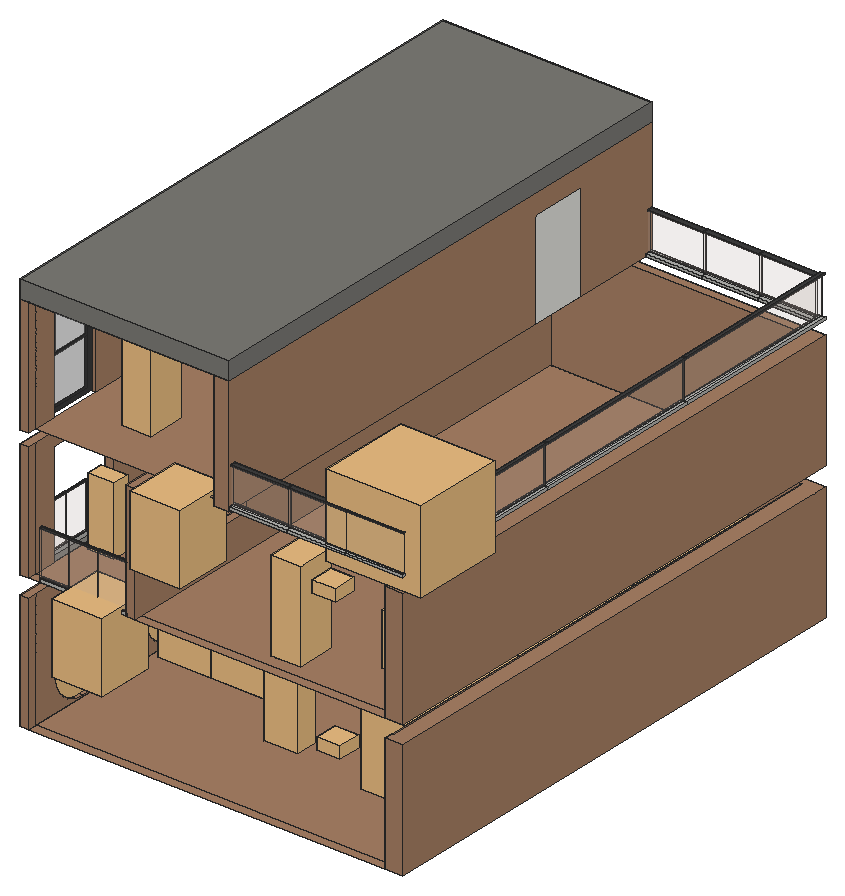
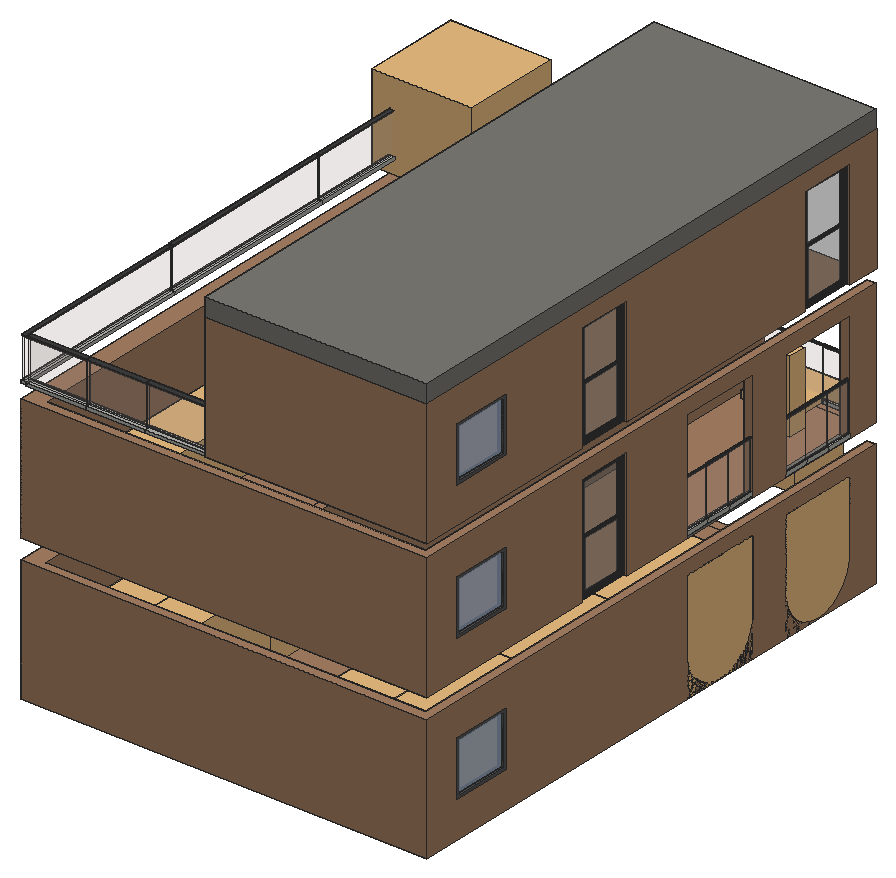
# SketchUp Ruby script. Lengths in inches.
U = 1.inch
M = Sketchup.active_model
def pt(a) = Geom::Point3d.new(a.map { |v| v * U })
def face(e, loops, mat)
  f = e.add_face(loops[0].map { |a| pt(a) })
  loops[1..].each { |l| e.add_face(l.map { |a| pt(a) }).erase! }
  f.material = f.back_material = mat if mat
  f
end
# faces: each face lists its corners as indices into pts; further lists are holes
def faces(e, pts, list, mat = nil) = list.each { |f| face(e, (f[0].is_a?(Array) ? f : [f]).map { |l| l.map { |i| pts[i] } }, mat) }
# xy, xz, yz: faces in a plane at the given z, y or x. An outline is a flat list of corners, or four numbers for a rectangle; further outlines are holes
def ring(l) = l.size == 4 ? [[l[0], l[1]], [l[2], l[1]], [l[2], l[3]], [l[0], l[3]]] : l.each_slice(2).to_a
def flat(e, list, mat, &to3) = list.each { |f| face(e, (f[0].is_a?(Array) ? f : [f]).map { |l| ring(l).map { |u, v| to3.(u, v) } }, mat) }
def xy(e, z, list, mat = nil) = flat(e, list, mat) { |x, y| [x, y, z] }
def xz(e, y, list, mat = nil) = flat(e, list, mat) { |x, z| [x, y, z] }
def yz(e, x, list, mat = nil) = flat(e, list, mat) { |y, z| [x, y, z] }
def lines(e, pts, list) = list.each { |a, b| e.add_line(pt(pts[a]), pt(pts[b])) }
# prism: a flat outline (further loops are holes) pulled along v
def prism(e, loops, v, mat = nil)
  f = face(e, loops, mat); d = Geom::Vector3d.new(v.map { |x| x * U })
  f.pushpull(f.normal.samedirection?(d) ? d.length : -d.length)
end
def box(e, o, s, mat = nil) = prism(e, [[o, [o[0] + s[0], o[1], o[2]], [o[0] + s[0], o[1] + s[1], o[2]], [o[0], o[1] + s[1], o[2]]]], [0, 0, s[2]], mat)
def at(x, y, z, deg = 0) = Geom::Transformation.translation(pt([x, y, z])) * Geom::Transformation.rotation(ORIGIN, Z_AXIS, deg.degrees)
def axes(o, x, y, z) = Geom::Transformation.new([*x, 0, *y, 0, *z, 0, *pt(o).to_a, 1])
def part(name) = M.definitions.add(name)
# library, detail: a bought-in or finely detailed component or shape, given as its bounding box
def library(name, o, s) = part(name).tap { |d| box(d.entities, o, s) }
def detail(e, o, s) = box(e.add_group.entities, o, s)
def put(e, d, t, mat = nil) = e.add_instance(d, t).tap { |i| i.material = mat if mat }
def group(e, t, mat = nil) = e.add_group.tap { |g| g.transformation = t; g.material = mat if mat }.entities
root = M.entities
M.materials.add("Aluminum_Anodized_Clear\#1").color = [178, 178, 174]
M.materials.add("Aluminum_Anodized_DarkGray\#1").color = [63, 63, 63]
M.materials.add("Bricks A04 100cm").color = [167, 128, 100]
M.materials.add("Concrete Grey 06 100cm").color = [123, 122, 117]
M.materials.add("Windows").color = [58, 58, 58]
M.materials.add("[Color_006]").color = [86, 86, 86]
M.materials.add("[Translucent Glass Gray]1").color = [128, 128, 128]
M.materials["[Translucent Glass Gray]1"].alpha = 0.5
M.materials.add("[Translucent_Glass_Gray]").color = [128, 128, 128]
M.materials["[Translucent_Glass_Gray]"].alpha = 0.5
M.materials.add("[Translucent_Glass_Gray]1").color = [167, 187, 214]
M.materials["[Translucent_Glass_Gray]1"].alpha = 0.8
M.materials.add("glass_architectural\#1").color = [217, 197, 188]
M.materials["glass_architectural\#1"].alpha = 0.1
c1 = library("Tariq 001 Standing",[-13.52,-8.8,0],[27.07,17.52,69.71])
c2 = library("Group\#170",[0,0,-0.09],[44.81,94.49,48.85])
c3 = library("Group\#172",[0,0,-0.09],[44.81,94.49,48.85])
c4 = part("Office workstation bank")
put(c4.entities,c2,at(188.98,44.81,0.09,-90))
put(c4.entities,c3,axes([0,44.81,0.09],[0,1,0],[1,0,0],[0,0,1]))
put(c4.entities,c3,axes([188.98,44.81,0.09],[0,1,0],[1,0,0],[0,0,1]))
put(c4.entities,c2,at(0,44.81,0.09,-90))
put(c4.entities,c2,at(94.49,44.81,0.09,-90))
put(c4.entities,c3,axes([94.49,44.81,0.09],[0,1,0],[1,0,0],[0,0,1]))
c5 = library("Group\#17",[0,0,0],[177.17,118.11,3.9375])
c6 = part("window+1")
g1 = group(c6.entities,at(0,0,177.17))
put(g1,c5,axes([0,0,0],[0,0,-1],[0,1,0],[1,0,0]))
g2 = group(g1,at(1.97,3.9375,-4.36),"[Translucent_Glass_Gray]")
yz(g2,0,[[0,-168.87,26.65,-142.34],[28.62,-168.87,51.08,-142.34],[59.15,-168.87,81.32,-142.34],[83.29,-168.87,110.24,-142.34],[0,-140.375,26.65,-114.83],
  [28.62,-140.375,51.08,-114.83],[59.15,-140.375,81.32,-114.83],[83.29,-140.375,110.24,-114.83],[0,-112.86,26.65,-87.32],[28.62,-112.86,51.08,-87.32],
  [59.15,-112.86,81.32,-87.32],[83.29,-112.86,110.24,-87.32],[0,-85.35,26.65,-58.83],[28.62,-85.35,51.08,-58.83],[59.15,-85.35,81.32,-58.83],
  [83.29,-85.35,110.24,-58.83],[0.55,-50.76,26.65,-50.76,26.93,-47.45,27.62,-44.2,28.72,-41.07,30.21,-38.1,32.07,-35.35,33.61,-33.59,15.58,-16.55,15.5625,-16.53,7.41,-27.15,1.91,-40.4375],[28.79,-50.76,52.17,-50.76,52.17,-27.38,50.2,-27.38,49.14,-27.47,46.14,-28.11,43.24,-29.125,40.5,-30.5,37.96,-32.22,35.65,-34.25,33.63,-36.55,31.91,-39.1,30.53,-41.84,29.52,-44.73,28.875,-47.74,28.79,-48.79],[58.07,-50.76,81.32,-50.76,81.32,-48.79,81.24,-47.74,80.61,-44.75,79.6,-41.87,78.24,-39.14,76.53,-36.61,74.52,-34.3125,72.22,-32.3,69.6875,-30.59,66.96,-29.22,64.08,-28.22,61.09,-27.59,60.04,-27.51,58.07,-27.51],[83.45,-50.76,109.68,-50.76,108.33,-40.4375,102.82,-27.15,94.67,-16.53,76.5625,-33.66,78.09,-35.4,79.94,-38.15,81.42,-41.1,82.51,-44.23,83.19,-47.46],
  [75.17,-32.27,93.28,-15.14,82.66,-6.99,69.375,-1.49,58.07,0,58.07,-25.38,61.37,-25.64,64.6,-26.32,67.73,-27.41,70.68,-28.89,73.43,-30.74],[35,-32.2,36.75,-30.66,39.51,-28.8,42.47,-27.31,45.61,-26.21,48.86,-25.52,52.17,-25.25,52.17,0,40.86,-1.49,27.58,-6.99,16.96,-15.14]])
put(g1,c5,axes([0,182.58,0],[0,0,-1],[0,1,0],[1,0,0]))
c7 = part("BIC_Bike Shop - Window - Small")
xy(c7.entities,-8,[[[0,0,36,36],[2,2,34,34]]],"[Color_006]")
xy(c7.entities,-4,[[2,2,34,34]],"[Translucent_Glass_Gray]1")
xy(c7.entities,0,[[[0,0,36,36],[2,2,34,34]]],"[Color_006]")
xz(c7.entities,0,[[0,-8,36,0]],"[Color_006]")
xz(c7.entities,2,[[2,-8,34,-4],[2,-4,34,0]],"[Color_006]")
xz(c7.entities,34,[[2,-8,34,-4],[2,-4,34,0]],"[Color_006]")
xz(c7.entities,36,[[0,-8,36,0]],"[Color_006]")
yz(c7.entities,0,[[0,-8,36,0]],"[Color_006]")
yz(c7.entities,2,[[2,-8,34,-4],[2,-4,34,0]],"[Color_006]")
yz(c7.entities,34,[[2,-8,34,-4],[2,-4,34,0]],"[Color_006]")
yz(c7.entities,36,[[0,-8,36,0]],"[Color_006]")
c8 = library("Untitled+(35)",[-36.2,-34.81,25.37],[51.5,58.42,71.3])
c9 = library("Dome Light",[-12,-12,0],[24,24,12])
c10 = part("Window+06")
g3 = group(c10.entities,at(-11,5.5,0,-90))
xy(g3,0,[[0,11,5.5,35]],"Windows")
xy(g3,2,[[0,13,5.5,33]],"Windows")
xy(g3,53,[[0,13,5.5,33]],"Windows")
xy(g3,55,[[0,11,5.5,35]],"Windows")
xz(g3,11,[[0,0,5.5,55]],"Windows")
xz(g3,13,[[0,2,5.5,53]],"Windows")
xz(g3,33,[[0,2,5.5,53]],"Windows")
xz(g3,35,[[0,0,5.5,55]],"Windows")
yz(g3,0,[[[11,0,35,55],[13,2,33,53]]],"Windows")
yz(g3,5.5,[[[11,0,35,55],[13,2,33,53]]],"Windows")
g4 = group(g3,at(2.75,2,2))
xy(g4,0,[[0,11,2,31]],"Windows")
xy(g4,1,[[0,12,1,30],[1,12,2,30]],"Windows")
xy(g4,25,[[0,12,1,30],[1,12,2,30]],"Windows")
xy(g4,26,[[0,11,2,31]],"Windows")
xz(g4,11,[[0,0,2,26]],"Windows")
xz(g4,12,[[0,1,1,25],[1,1,2,25]],"Windows")
xz(g4,30,[[0,1,1,25],[1,1,2,25]],"Windows")
xz(g4,31,[[0,0,2,26]],"Windows")
yz(g4,0,[[[11,0,31,26],[12,1,30,25]]],"Windows")
yz(g4,1,[[12,1,30,25]],"[Translucent Glass Gray]1")
yz(g4,2,[[[11,0,31,26],[12,1,30,25]]],"Windows")
g5 = group(g3,at(0.75,2,27))
xy(g5,0,[[0,11,2,31]],"Windows")
xy(g5,1,[[0,12,1,30],[1,12,2,30]],"Windows")
xy(g5,25,[[0,12,1,30],[1,12,2,30]],"Windows")
xy(g5,26,[[0,11,2,31]],"Windows")
xz(g5,11,[[0,0,2,26]],"Windows")
xz(g5,12,[[0,1,1,25],[1,1,2,25]],"Windows")
xz(g5,30,[[0,1,1,25],[1,1,2,25]],"Windows")
xz(g5,31,[[0,0,2,26]],"Windows")
yz(g5,0,[[[11,0,31,26],[12,1,30,25]]],"Windows")
yz(g5,1,[[12,1,30,25]],"[Translucent Glass Gray]1")
yz(g5,2,[[[11,0,31,26],[12,1,30,25]]],"Windows")
c11 = library("Reception desk",[23.57,0,0],[37.45,80.71,54.72])
c12 = library("Katja 001 Standing",[-10.51,-13.65,0],[20.97,27.3,64.32])
c13 = part("GLASS")
prism(c13.entities,[[[48,0,0],[0,0,0],[0,0.8,0],[48.96,0.8,0]]],[0,0,36])
c14 = part("STEEL BAR")
box(c14.entities,[0,-0.1,0],[48,1.8,1.2])
c15 = part("LOWER PART")
box(c15.entities,[0,-0.6,0],[48.6,2.6,2.6])
c16 = part("BALCONY GLASS ")
put(c16.entities,c13,at(0,0.9,2.6),"glass_architectural\#1")
put(c16.entities,c14,at(0,0.5,38.6),"Aluminum_Anodized_DarkGray\#1")
put(c16.entities,c15,at(0,0.6,0),"Aluminum_Anodized_Clear\#1")
c17 = part("NO 3")
put(c17.entities,c16,at(0,0,0))
put(c17.entities,c16,at(48.6,0,0))
put(c17.entities,c16,at(97.2,0,0))
c18 = library("Dome Light\#1",[-12,-12,0],[24,24,12])
c19 = library("Palmilla",[-52.93,-43.2,-6.65],[96.66,94.88,84.22])
box(root,[396.25,532.6875,414.5625],[57.5625,56.26,98.76])
xy(root,281.8125,[[240.0625,289.51,249.0625,368.7]])
xy(root,282.82,[[240.0625,173.32,249.0625,249.35]],"Concrete Grey 06 100cm")
xy(root,283.0625,[[240.0625,289.51,249.0625,368.7]])
xz(root,289.51,[[240.0625,281.8125,249.0625,283.0625]])
xz(root,368.7,[[240.0625,281.8125,249.0625,283.0625]])
yz(root,240.0625,[[173.32,281.8125,173.32,282.82,249.35,282.82,252.52,281.8125],[289.51,281.8125,368.7,283.0625]],"Concrete Grey 06 100cm")
yz(root,249.0625,[[289.51,281.8125,368.7,283.0625]])
put(root,c1,axes([423.48,256.09,142.06],[1.25,0,0],[0,1.25,0],[0,0,1.25]))
put(root,c4,axes([516.21,672.11,142.85],[0,-1.55368,0],[1,0,0],[0,0,1.5]))
put(root,c4,axes([255.82,645.9,142.9375],[0,-1.22741,0],[1.21,0,0],[0,0,1.89]))
g6 = group(root,at(-660.5625,139.09,152))
xy(g6,-9.0625,[[900.625,2.02,900.625,542.02,1292.125,542.02,1292.125,2.02,1273.39,2.02,1273.39,11.02,1274.625,11.02,1274.625,533.02,909.625,533.02,909.625,2.02],[909.625,2.02,1273.39,11.02],[909.625,11.02,1274.625,533.02]],"Bricks A04 100cm")
xy(g6,25.83,[[900.625,446.52,909.625,507.83]],"Bricks A04 100cm")
xy(g6,79.86,[[900.625,446.52,909.625,507.83]],"Bricks A04 100cm")
xy(g6,97.8125,[[900.625,34.24,909.625,110.61],[900.625,149.74,909.625,229.61]],"Bricks A04 100cm")
xy(g6,110.9375,[[900.625,2.02,909.625,2.02,909.625,533.02,1274.625,533.02,1274.625,11.02,1273.39,11.02,1273.39,2.02,1292.125,2.02,1292.125,542.02,900.625,542.02]],"Bricks A04 100cm")
xy(g6,129.8125,[[1273.125,2.02,1273.125,11.02,1273,11.02,1273,533.02,909.625,533.02,909.625,355.8,900.625,355.8,900.625,542.02,1292.125,542.02,1292.125,2.02],[900.625,2.02,909.625,34.24],[909.625,2.02,1004.08,11.02],[1004.08,2.02,1009.14,11.02],[1018.32,2.02,1273.125,11.02],
  [909.625,11.02,1009.14,533.02],[1018.32,11.02,1273,533.02],[900.625,110.61,909.625,150.42],[900.625,229.61,909.625,302.3]],"Bricks A04 100cm")
xy(g6,164.58,[[900.625,446.52,909.625,507.83]],"Bricks A04 100cm")
xy(g6,165.37,[[1009.14,74.68,1018.32,144.86]],"Bricks A04 100cm")
xy(g6,208.74,[[1009.14,74.68,1018.32,144.86]],"Bricks A04 100cm")
xy(g6,218.61,[[900.625,446.52,909.625,507.83]],"Bricks A04 100cm")
xy(g6,235.875,[[900.625,34.24,909.625,110.61],[900.625,150.42,909.625,229.61],[900.625,302.3,909.625,355.8]],"Bricks A04 100cm")
xy(g6,249.8125,[[900.625,2.02,909.625,2.02,909.625,533.02,1273,533.02,1273,11.02,1273.125,11.02,1273.125,2.02,1292.125,2.02,1292.125,542.02,900.625,542.02],[1009.14,2.02,1018.32,533.02]],"Bricks A04 100cm")
xz(g6,2.02,[[900.625,-9.0625,909.625,110.9375],[1273.39,-9.0625,1292.125,110.9375],[900.625,129.8125,909.625,249.8125],[1009.14,129.8125,1018.32,249.8125],[1273.125,129.8125,1292.125,249.8125]],"Bricks A04 100cm")
xz(g6,11.02,[[1273.39,-9.0625,1274.625,110.9375],[1273,129.8125,1273.125,249.8125]],"Bricks A04 100cm")
xz(g6,34.24,[[900.625,25.1875,909.625,39],[900.625,39,909.625,97.8125],[900.625,129.8125,909.625,235.875]],"Bricks A04 100cm")
xz(g6,74.68,[[1009.14,165.37,1018.32,208.74]],"Bricks A04 100cm")
xz(g6,110.61,[[900.625,25.1875,909.625,39],[900.625,39,909.625,97.8125],[900.625,129.8125,909.625,235.875]],"Bricks A04 100cm")
xz(g6,144.86,[[1009.14,165.37,1018.32,208.74]],"Bricks A04 100cm")
xz(g6,149.74,[[900.625,25.1875,909.625,39],[900.625,39,909.625,97.8125]],"Bricks A04 100cm")
xz(g6,150.42,[[900.625,129.8125,909.625,235.875]],"Bricks A04 100cm")
xz(g6,229.61,[[900.625,25.1875,909.625,39],[900.625,39,909.625,97.8125],[900.625,129.8125,909.625,235.875]],"Bricks A04 100cm")
xz(g6,302.3,[[900.625,129.8125,909.625,235.875]],"Bricks A04 100cm")
xz(g6,355.8,[[900.625,129.8125,909.625,235.875]],"Bricks A04 100cm")
xz(g6,446.52,[[900.625,25.83,909.625,79.86],[900.625,164.58,909.625,218.61]],"Bricks A04 100cm")
xz(g6,507.83,[[900.625,25.83,909.625,79.86],[900.625,164.58,909.625,218.61]],"Bricks A04 100cm")
xz(g6,533.02,[[909.625,-9.0625,1274.625,110.9375],[909.625,129.8125,1009.14,249.8125],[1009.14,129.8125,1018.32,249.8125],[1018.32,129.8125,1273,249.8125]],"Bricks A04 100cm")
xz(g6,542.02,[[900.625,-9.0625,1292.125,110.9375],[900.625,129.8125,1292.125,249.8125]],"Bricks A04 100cm")
yz(g6,900.625,[[[2.02,-9.0625,542.02,110.9375],[189.67,-8.5625,199.0625,-7.46,207.9375,-4.21,215.82,1,222.28,7.91,226.96,16.12,229.61,25.1875,229.61,97.8125,149.74,97.8125,149.74,25.1875,152.39,16.12,157.07,7.91,163.53,1,171.41,-4.21,180.29,-7.46],[72.42,-8.5625,81.62,-7.45,90.28,-4.17,97.91,1.08,104.06,8.01,108.375,16.2,110.61,25.1875,110.61,97.8125,34.24,97.8125,34.24,25.1875,36.47,16.2,40.79,8.01,46.94,1.08,54.57,-4.17,63.23,-7.45],[446.52,25.83,507.83,79.86]],[[2.02,129.8125,2.02,249.8125,542.02,249.8125,542.02,129.8125,355.8,129.8125,355.8,235.875,302.3,235.875,302.3,129.8125,229.61,129.8125,229.61,235.875,150.42,235.875,150.42,129.8125,110.61,129.8125,110.61,235.875,34.24,235.875,34.24,129.8125],[446.52,164.58,507.83,218.61]]],"Bricks A04 100cm")
yz(g6,909.625,[[2.02,-9.0625,11.02,110.9375],[[11.02,-9.0625,533.02,110.9375],[189.67,-8.5625,180.29,-7.46,171.41,-4.21,163.53,1,157.07,7.91,152.39,16.12,149.74,25.1875,149.74,97.8125,229.61,97.8125,229.61,25.1875,226.96,16.12,222.28,7.91,215.82,1,207.9375,-4.21,199.0625,-7.46],[72.42,-8.5625,63.23,-7.45,54.57,-4.17,46.94,1.08,40.79,8.01,36.47,16.2,34.24,25.1875,34.24,97.8125,110.61,97.8125,110.61,25.1875,108.375,16.2,104.06,8.01,97.91,1.08,90.28,-4.17,81.62,-7.45],[446.52,25.83,507.83,79.86]],[2.02,129.8125,11.02,249.8125],[[11.02,129.8125,34.24,129.8125,34.24,235.875,110.61,235.875,110.61,129.8125,150.42,129.8125,150.42,235.875,229.61,235.875,229.61,129.8125,302.3,129.8125,302.3,235.875,355.8,235.875,355.8,129.8125,533.02,129.8125,533.02,249.8125,11.02,249.8125],[446.52,164.58,507.83,218.61]]],"Bricks A04 100cm")
yz(g6,1009.14,[[[2.02,129.8125,533.02,249.8125],[74.68,165.37,144.86,208.74]]],"Bricks A04 100cm")
yz(g6,1018.32,[[[2.02,129.8125,533.02,249.8125],[74.68,165.37,144.86,208.74]]],"Bricks A04 100cm")
yz(g6,1273,[[11.02,129.8125,533.02,249.8125]],"Bricks A04 100cm")
yz(g6,1273.125,[[2.02,129.8125,11.02,249.8125]],"Bricks A04 100cm")
yz(g6,1273.39,[[2.02,-9.0625,11.02,110.9375]],"Bricks A04 100cm")
yz(g6,1274.625,[[11.02,-9.0625,533.02,110.9375]],"Bricks A04 100cm")
yz(g6,1292.125,[[2.02,-9.0625,542.02,110.9375],[2.02,129.8125,542.02,249.8125]],"Bricks A04 100cm")
p = [[900.625,72.42,-8.5625],[900.625,63.23,-7.45],[909.625,63.23,-7.45],[909.625,72.42,-8.5625],[900.625,81.62,-7.45],[909.625,81.62,-7.45],
  [900.625,189.67,-8.5625],[900.625,180.29,-7.46],[909.625,180.29,-7.46],[909.625,189.67,-8.5625],[900.625,199.0625,-7.46],[909.625,199.0625,-7.46],
  [900.625,171.41,-4.21],[909.625,171.41,-4.21],[900.625,207.9375,-4.21],[909.625,207.9375,-4.21],[900.625,54.57,-4.17],[909.625,54.57,-4.17],
  [900.625,90.28,-4.17],[909.625,90.28,-4.17],[900.625,46.94,1.08],[909.625,46.94,1.08],[900.625,97.91,1.08],[909.625,97.91,1.08],
  [900.625,163.53,1],[909.625,163.53,1],[900.625,215.82,1],[909.625,215.82,1],[900.625,157.07,7.91],[909.625,157.07,7.91],
  [900.625,222.28,7.91],[909.625,222.28,7.91],[900.625,40.79,8.01],[909.625,40.79,8.01],[900.625,104.06,8.01],[909.625,104.06,8.01],
  [900.625,152.39,16.12],[909.625,152.39,16.12],[900.625,226.96,16.12],[909.625,226.96,16.12],[900.625,36.47,16.2],[909.625,36.47,16.2],
  [900.625,108.375,16.2],[909.625,108.375,16.2],[900.625,149.74,25.1875],[909.625,149.74,25.1875],[900.625,229.61,25.1875],[909.625,229.61,25.1875],
  [900.625,34.24,25.1875],[909.625,34.24,25.1875],[900.625,110.61,25.1875],[909.625,110.61,25.1875]]
faces(g6,p,[[0,1,2,3],[4,0,3,5],[6,7,8,9],[10,6,9,11],[7,12,13,8],[14,10,11,15],[1,16,17,2],[18,4,5,19],
  [16,20,21,17],[22,18,19,23],[12,24,25,13],[26,14,15,27],[24,28,29,25],[30,26,27,31],[20,32,33,21],[34,22,23,35],
  [28,36,37,29],[38,30,31,39],[32,40,41,33],[42,34,35,43],[36,44,45,37],[46,38,39,47],[40,48,49,41],[50,42,43,51]],"Bricks A04 100cm")
put(root,c6,axes([244,173.32,249.8125],[-1,0,0],[0,0.64664,0],[0,0,-0.60043]))
put(root,c7,axes([240.0625,646.92,177.83],[0,-1.70312,0],[0,0,1.50107],[-0.5763,0,0]))
put(root,c8,at(327.84,151.59,191.76))
put(root,c9,at(560.9,145.76,232.72))
put(root,c10,axes([242.3125,494.89,281.8125],[0,-2.22917,0],[0.375,0,0],[0,0,1.92841]))
put(root,c11,axes([526.98,465.16,281.8125],[1.39,0,0],[0,2.085,0],[0,0,0.96744]))
put(root,c11,axes([526.98,203.22,281.8125],[1.39,0,0],[0,2.085,0],[0,0,0.96744]))
put(root,c12,axes([493.89,183.04,281.8125],[1.43,0,0],[0,1.43,0],[0,0,1.43]))
put(root,c17,axes([348.8125,143.71,281.8125],[-0.60765,0,0],[0,-1,0],[0,0,1.27]))
put(root,c17,axes([242.66,173.32,282.82],[0,0.52383,0],[-1,0,0],[0,0,1.27]))
put(root,c17,axes([243.98,289.51,283.0625],[0,0.54268,0],[-1,0,0],[0,0,1.27]))
put(root,c1,at(279.875,203.41,291.03))
put(root,c7,axes([240.0625,646.92,316.58],[0,-1.70312,0],[0,0,1.50107],[-0.5763,0,0]))
put(root,c8,at(410.95,147.59,321.35))
put(root,c18,at(560.23,140.88,378.76))
put(root,c19,at(604.06,186.73,408.9))
put(root,c17,axes([625.98,681.11,414.5625],[-1.177,0,0],[0,-3.0602,0],[0,0,1.07]))
put(root,c10,axes([242.3125,494.89,414.5625],[0,-2.22917,0],[0.375,0,0],[0,0,1.92841]))
put(root,c10,axes([242.5,226.82,414.5625],[0,-2.22917,0],[0.375,0,0],[0,0,1.92841]))
put(root,c12,axes([313.79,216.76,414.5625],[1.43,0,0],[0,1.43,0],[0,0,1.43]))
g7 = group(root,at(-656.73,139.09,410))
xy(g7,4.5625,[[896.79,2.02,905.79,34.24],[1094.55,2.08,1094.55,533.02,905.79,533.02,905.79,355.8,896.79,355.8,896.79,542.02,1110.54,542.02,1110.54,2.08],[905.79,11.02,1094.55,533.02],[896.79,87.86,905.79,302.3]],"Bricks A04 100cm")
xy(g7,38.7,[[896.79,446.52,905.79,507.83]],"Bricks A04 100cm")
xy(g7,92.74,[[896.79,446.52,905.79,507.83]],"Bricks A04 100cm")
xy(g7,108.5,[[896.79,34.24,905.79,87.86],[896.79,302.3,905.79,355.8]],"Bricks A04 100cm")
xy(g7,124.5625,[[896.79,2.02,905.79,2.02,905.79,533.02,1094.55,533.02,1094.55,2.08,1110.54,2.08,1110.54,542.02,896.79,542.02]],"Bricks A04 100cm")
xz(g7,2.02,[[896.79,4.5625,905.79,124.5625]],"Bricks A04 100cm")
xz(g7,2.08,[[1094.55,4.5625,1110.54,124.5625]],"Bricks A04 100cm")
xz(g7,34.24,[[896.79,4.5625,905.79,108.5]],"Bricks A04 100cm")
xz(g7,87.86,[[896.79,4.5625,905.79,108.5]],"Bricks A04 100cm")
xz(g7,302.3,[[896.79,4.5625,905.79,108.5]],"Bricks A04 100cm")
xz(g7,355.8,[[896.79,4.5625,905.79,108.5]],"Bricks A04 100cm")
xz(g7,446.52,[[896.79,38.7,905.79,92.74]],"Bricks A04 100cm")
xz(g7,507.83,[[896.79,38.7,905.79,92.74]],"Bricks A04 100cm")
xz(g7,533.02,[[905.79,4.5625,1094.55,124.5625]],"Bricks A04 100cm")
xz(g7,542.02,[[896.79,4.5625,1110.54,124.5625]],"Bricks A04 100cm")
yz(g7,896.79,[[[2.02,4.5625,2.02,124.5625,542.02,124.5625,542.02,4.5625,355.8,4.5625,355.8,108.5,302.3,108.5,302.3,4.5625,87.86,4.5625,87.86,108.5,34.24,108.5,34.24,4.5625],[446.52,38.7,507.83,92.74]]],"Bricks A04 100cm")
yz(g7,905.79,[[2.02,4.5625,11.02,124.5625],[[11.02,4.5625,34.24,4.5625,34.24,108.5,87.86,108.5,87.86,4.5625,302.3,4.5625,302.3,108.5,355.8,108.5,355.8,4.5625,533.02,4.5625,533.02,124.5625,11.02,124.5625],[446.52,38.7,507.83,92.74]]],"Bricks A04 100cm")
yz(g7,1094.55,[[2.08,4.5625,533.02,124.5625]],"Bricks A04 100cm")
yz(g7,1110.54,[[2.08,4.5625,542.02,124.5625]],"Bricks A04 100cm")
put(root,c17,axes([625.3,680.71,415.51],[0,-3.6487,0],[2.4075,0,0],[0,0,1.07]))
put(root,c17,axes([631.5625,148.73,416.25],[-1.21914,0,0],[0,-3.0602,0],[0,0,1.0272]))
put(root,c7,axes([240.0625,646.92,448.7],[0,-1.70312,0],[0,0,1.50107],[-0.5763,0,0]))
g8 = group(root,at(-660.5625,139.09,531.125))
g9 = group(g8,at(315.95,2.02,-23.99))
box(g9,[584.68,0,27.43],[213.75,540,17.62],"Concrete Grey 06 100cm")
